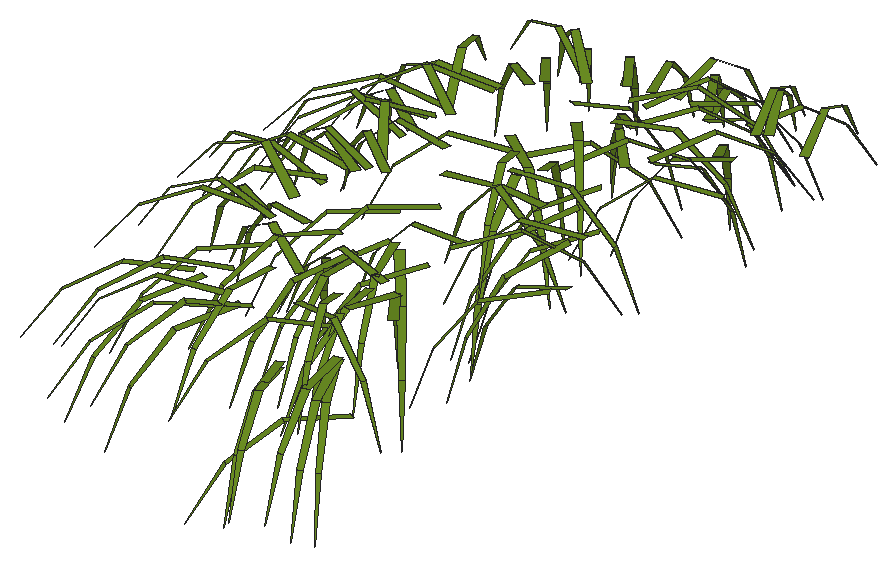
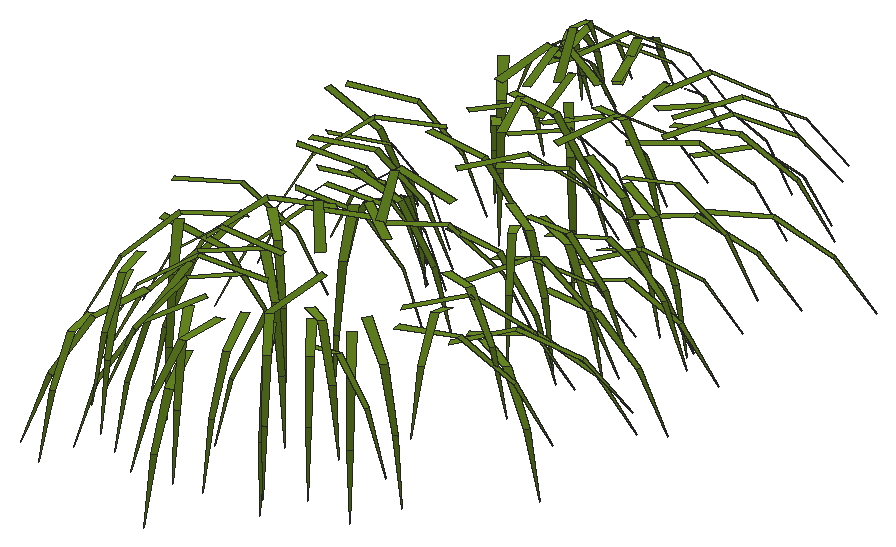
# SketchUp Ruby script. Lengths in inches.
U = 1.inch
M = Sketchup.active_model
def pt(a) = Geom::Point3d.new(a.map { |v| v * U })
def face(e, loops, mat)
  f = e.add_face(loops[0].map { |a| pt(a) })
  loops[1..].each { |l| e.add_face(l.map { |a| pt(a) }).erase! }
  f.material = f.back_material = mat if mat
  f
end
# faces: each face lists its corners as indices into pts; further lists are holes
def faces(e, pts, list, mat = nil) = list.each { |f| face(e, (f[0].is_a?(Array) ? f : [f]).map { |l| l.map { |i| pts[i] } }, mat) }
# xy, xz, yz: faces in a plane at the given z, y or x. An outline is a flat list of corners, or four numbers for a rectangle; further outlines are holes
def ring(l) = l.size == 4 ? [[l[0], l[1]], [l[2], l[1]], [l[2], l[3]], [l[0], l[3]]] : l.each_slice(2).to_a
def flat(e, list, mat, &to3) = list.each { |f| face(e, (f[0].is_a?(Array) ? f : [f]).map { |l| ring(l).map { |u, v| to3.(u, v) } }, mat) }
def xy(e, z, list, mat = nil) = flat(e, list, mat) { |x, y| [x, y, z] }
def xz(e, y, list, mat = nil) = flat(e, list, mat) { |x, z| [x, y, z] }
def yz(e, x, list, mat = nil) = flat(e, list, mat) { |y, z| [x, y, z] }
def lines(e, pts, list) = list.each { |a, b| e.add_line(pt(pts[a]), pt(pts[b])) }
# prism: a flat outline (further loops are holes) pulled along v
def prism(e, loops, v, mat = nil)
  f = face(e, loops, mat); d = Geom::Vector3d.new(v.map { |x| x * U })
  f.pushpull(f.normal.samedirection?(d) ? d.length : -d.length)
end
def box(e, o, s, mat = nil) = prism(e, [[o, [o[0] + s[0], o[1], o[2]], [o[0] + s[0], o[1] + s[1], o[2]], [o[0], o[1] + s[1], o[2]]]], [0, 0, s[2]], mat)
def at(x, y, z, deg = 0) = Geom::Transformation.translation(pt([x, y, z])) * Geom::Transformation.rotation(ORIGIN, Z_AXIS, deg.degrees)
def axes(o, x, y, z) = Geom::Transformation.new([*x, 0, *y, 0, *z, 0, *pt(o).to_a, 1])
def part(name) = M.definitions.add(name)
# library, detail: a bought-in or finely detailed component or shape, given as its bounding box
def library(name, o, s) = part(name).tap { |d| box(d.entities, o, s) }
def detail(e, o, s) = box(e.add_group.entities, o, s)
def put(e, d, t, mat = nil) = e.add_instance(d, t).tap { |i| i.material = mat if mat }
def group(e, t, mat = nil) = e.add_group.tap { |g| g.transformation = t; g.material = mat if mat }.entities
root = M.entities
M.materials.add("[0061_OliveDrab]").color = [107, 142, 35]
p = [[558.84,17.43,556.17],[558.64,17.37,556.17],[558.94,16.75,553.64],[561.49,28.35,556.17],[561.67,28.32,556.17],[561.7,29.01,553.63],
  [560.05,32.29,556.14],[560.24,32.3,556.14],[560.12,33.01,553.61],[556.33,35.38,555.85],[556.52,35.47,555.85],[555.86,36.71,553.64],
  [557.52,19.82,556.28],[557.4,20,556.28],[556.89,19.5,553.75],[556.22,25.11,556.28],[556.39,25.21,556.28],[555.97,25.77,553.75],
  [560.34,11.25,556.31],[560.17,11.11,556.31],[560.71,10.64,553.78],[560.23,14.95,556.35],[560.0625,15.05,556.35],[559.76,14.39,553.83],
  [557.125,30.02,556.3],[557.3,29.96,556.3],[557.46,30.66,553.77],[550.61,31.32,556.24],[550.78,31.45,556.24],[550.13,32.12,553.78],
  [562.33,3.99,556.375],[562.16,3.89,556.375],[562.74,3.09,553.94],[553.13,4.65,556.38],[552.93,4.75,556.38],[552.59,3.82,553.95],
  [550.63,5.69,556.26],[550.45,5.77,556.26],[550.1,4.65,553.91],[546.34,9.17,556],[546.24,9.36,556],[544.9375,8.58,553.86],
  [558.5,17.37,556.38],[558.33,17.5,556.38],[557.95,16.85,553.87],[559.33,17.32,556.42],[559.21,17.49,556.42],[558.65,16.99,553.91],
  [560.17,29.72,556.41],[560.34,29.83,556.41],[559.85,30.39,553.89],[553.38,32.92,556.3125],[553.55,33.04,556.3125],[552.94,33.75,553.86],
  [554.14,14.23,556.52],[554.29,14.37,556.52],[553.72,14.88,554.01],[560.3,15.8,556.48],[560.3125,15.99,556.48],[559.55,15.94,553.96],
  [555.68,28.9,556.47],[555.8125,29.05,556.47],[555.2,29.48,553.95],[549.85,29.7,556.44],[549.97,29.87,556.44],[549.15,30.37,553.99],
  [560.62,33.35,556.43],[560.79,33.26,556.43],[561.13,34.09,553.96],[561.81,3.6,556.51],[561.59,3.52,556.51],[562.09,2.55,554.125],
  [559.3,2.32,556.41],[559.12,2.43,556.41],[558.46,1.07,554.26],[558.97,25.82,556.75],[558.9375,26.01,556.75],[558.15,25.76,554.26],
  [546.47,26.42,556.47],[546.58,26.6,556.47],[545.28,27.31,554.3],[560.37,12.8,556.88],[560.25,12.99,556.88],[559.59,12.45,554.4],
  [545.98,20.68,556.59],[546.01,20.875,556.59],[544.54,20.99,554.42],[549.97,15.21,556.95],[550.04,15.39,556.95],[549.18,15.63,554.48],
  [553.375,32.76,556.92],[553.53,32.88,556.92],[552.78,33.73,554.55],[555.23,9,557.05],[555.03,9.07,557.05],[554.81,8.19,554.58],
  [555.34,10.51,557.05],[555.17,10.6,557.05],[554.85,9.74,554.59],[558.125,13.4,557.08],[558.3,13.53,557.08],[557.67,14.18,554.62],
  [559.74,2.57,556.85],[559.56,2.5,556.85],[560.14,1.16,554.66],[548.14,15.86,557.11],[548.24,16.04,557.11],[547.28,16.4375,554.69],
  [551.95,32.03,557.04],[552.11,32.15,557.04],[551.38,32.95,554.65],[555.03,33.72,557.02],[555.2,33.8,557.02],[554.625,34.89,554.7],
  [556.47,33.9,556.98],[556.65,34.02,556.98],[555.875,35,554.67],[561.18,3.24,557.09],[560.97,3.2,557.09],[561.35,1.98,554.79],
  [561.63,34.73,556.97],[561.85,34.7,556.97],[561.95,36.12,554.76],[557.27,10.02,557.3],[557.09,10.11,557.3],[556.72,9.24,554.85],
  [555.47,20.5,557.35],[555.51,20.72,557.35],[554.55,20.78,554.91],[546.35,22.66,557.09],[546.28,22.84,557.09],[544.93,22.23,554.92],
  [550.36,8.76,557.39],[550.24,8.9,557.39],[549.45,8.05,555.03],[547.56,15.15,557.24],[547.41,15.31,557.24],[546.48,14.29,555],
  [555,16.09,557.47],[555.01,16.28,557.47],[554.02,16.24,555.04],[560.78,35.62,557.02],[560.95,35.6875,557.02],[560.26,37.17,554.97],
  [560.04,2.46,557.18],[559.84,2.38,557.18],[560.56,0.96,555.1],[552.52,13.61,557.52],[552.4,13.77,557.52],[551.65,13.07,555.1],
  [549.33,7.52,557.36],[549.26,7.72,557.36],[547.92,7.2,555.16],[556.98,34.77,557.55],[557.18,34.8,557.55],[556.91,36.14,555.3],
  [558.04,17.8,557.84],[557.99,18,557.84],[556.97,17.66,555.44],[559.38,20.45,557.84],[559.25,20.27,557.84],[560.16,19.74,555.43],
  [561.73,21.58,557.77],[561.75,21.39,557.77],[562.78,21.56,555.37],[549.97,21.59,557.79],[550.01,21.79,557.79],[548.93,21.86,555.39],
  [559.22,10.29,557.83],[559.05,10.22,557.83],[559.58,9.23,555.45],[548.57,20.19,557.86],[548.68,20.39,557.86],[547.57,20.875,555.52],
  [545.75,18.6,557.625],[545.75,18.81,557.625],[544.04,18.68,555.63],[547.52,25.83,557.72],[547.49,26.05,557.72],[545.97,25.71,555.61],
  [557.06,27.1,557.9375],[557.2,27.24,557.9375],[556.32,28.03,555.59],[559.71,33.8125,557.84],[559.88,33.91,557.84],[559.1,35.07,555.62],
  [551.48,4.44,557.76],[551.33,4.55,557.76],[550.46,3.25,555.65],[554.38,12.95,558.11],[554.43,13.15,558.11],[553.3,13.32,555.74],
  [550.11,20.86,558.08],[550.23,21.02,558.08],[549.26,21.6,555.7],[560.01,6.83,558.12],[559.82,6.79,558.12],[560.21,5.71,555.76],
  [546.625,13.15,557.81],[546.55,13.36,557.81],[545.04,12.7,555.76],[554.09,13.77,558.17],[553.93,13.9,558.17],[553.24,12.88,555.85],
  [552.38,20.5,558.18],[552.3,20.7,558.18],[551.26,20.17,555.82],[560.04,22.71,558.16],[559.98,22.9,558.16],[558.89,22.42,555.82],
  [557.14,33.43,557.4],[557.42,33.55,557.4],[553.1,4.48,558.14],[552.92,4.59,558.14],[552.28,3.41,555.89],[555.11,5.875,558.09],
  [554.92,5.87,558.09],[555.08,4.5,555.85],[560.17,19.36,558.28],[560.16,19.14,558.28],[561.33,19.2,555.92],[562.49,26.92,558.26],
  [562.52,26.72,558.26],[563.6875,26.98,555.92],[561.45,7.63,558.28],[561.38,7.46,558.28],[562.57,7.09,555.96],[548.34,10.13,557.41],
  [548.2,10.4,557.41],[547.29,17.83,558.18],[547.27,18.05,558.18],[545.88,17.8,555.96],[559.84,32.17,558.34],[560.02,32.09,558.34],
  [560.4375,33.27,556.03],[559.39,6.9,558.37],[559.17,6.92,558.37],[559.15,5.68,556.06],[546.47,23.29,557.99],[546.39,23.48,557.99],
  [544.8,22.66,556.07],[560.31,25.19,558.4],[560.45,25.03,558.4],[561.26,25.89,556.05],[561.15,30.25,558.34],[561.3125,30.14,558.34],
  [561.98,31.33,556.09],[560.08,30.88,558.35],[560.34,30.89,558.35],[558.48,18.75,558.42],[558.2,18.66,558.42],[561.21,27.02,558.41],
  [561.46,26.97,558.41],[551.62,29.95,558.24],[551.86,30.14,558.24],[551.53,31.18,558.53],[551.68,31.34,558.53],[550.66,32.09,556.22],
  [551.4,7.46,558.04],[551.13,7.57,558.04],[553.51,9.45,558.54],[553.32,9.54,558.54],[552.88,8.28,556.28],[559.47,12.37,558.52],
  [559.23,12.17,558.52],[561.01,16.15,558.55],[560.78,16.3,558.55],[548.38,19.6,558.47],[548.43,19.79,558.47],[547.01,20.1,556.28],
  [558.6875,20.6,558.5],[558.51,20.85,558.5],[556.87,23.87,558.5],[557.11,24,558.5],[556.6,28.7,558.5],[556.85,28.61,558.5],
  [554.31,31.49,558.3],[554.54,31.64,558.3],[560.48,4.26,557.74],[560.22,4.41,557.74],[561.48,5.55,558.31],[561.23,5.41,558.31],
  [553.96,6.21,558.32],[553.67,6.35,558.32],[550.17,6.52,558.46],[550,6.67,558.46],[549.01,5.375,556.41],[558,8.09,558.63],
  [557.82,8.05,558.63],[558.19,6.69,556.42],[547.51,13.85,558.54],[547.51,14.03,558.54],[545.97,14.02,556.42],[560.56,18.11,558.6],
  [560.4,18.35,558.6],[559.44,18.49,558.56],[559.2,18.67,558.56],[562.47,18.78,558.65],[562.6,18.64,558.65],[563.52,19.67,556.42],
  [546.41,18.67,558.32],[546.5,18.875,558.32],[544.84,19.49,556.38],[548.86,19.73,558.61],[548.72,19.87,558.61],[547.76,18.78,556.42],
  [548.42,23.68,558.57],[548.33,23.87,558.57],[547.05,23.11,556.4],[560.93,28.48,558.59],[561.17,28.64,558.59],[551.18,28.62,558.41],
  [551.36,28.85,558.41],[549.74,31.49,558.39],[549.82,31.66,558.39],[548.3,32.33,556.36],[559.8,31.89,558.46],[560.04,31.76,558.46],
  [556.64,4.64,558.67],[556.48,4.74,558.67],[555.79,3.49,556.46],[561.18,5.36,558.36],[560.88,5.25,558.36],[555.08,13.07,558.67],
  [555.3,13.26,558.67],[561.78,15.68,558.65],[561.79,15.95,558.65],[548.32,25.18,557.86],[548.48,25.43,557.86],[556.74,27.87,558.64],
  [556.93,28.07,558.64],[561.34,30.23,558.74],[561.44,30.03,558.74],[562.52,30.74,556.46],[560.22,33.36,558.59],[560.39,33.43,558.59],
  [559.67,34.88,556.53],[551.68,12.85,558.85],[551.78,13.04,558.85],[550.46,13.6,556.64],[548.16,20.32,558.01],[548.2,20.6,558.01],
  [547.57,21.51,558.76],[547.58,21.7,558.76],[546.16,21.73,556.55],[548.63,25.72,558.76],[548.74,25.89,558.76],[547.39,26.6,556.62],
  [563.01,29,558.79],[563.19,28.9,558.79],[563.82,30.2,556.6],[560.53,26.08,558.84],[560.48,26.35,558.84],[559.04,4.65,558.28],
  [558.78,4.56,558.28],[558.71,18.14,559.05],[558.53,18.06,559.05],[559.25,16.82,556.85],[560.13,21.67,558.93],[559.97,21.53,558.93],
  [561.02,20.46,556.77],[561.77,13.625,558.9375],[561.61,13.89,558.9375],[550.1,22.92,559.08],[550.28,23.05,559.08],[549.34,24.17,556.89],
  [561.24,26.37,559.06],[561.42,26.24,559.06],[562.19,27.55,556.92],[554.47,31.2,558.72],[554.7,31.37,558.72],[555.87,10.5625,559.05],
  [555.59,10.67,559.05],[551.51,14.55,558.97],[551.62,14.8125,558.97],[549.46,28.73,558.94],[549.64,28.82,558.94],[548.76,30.32,556.97],
  [553.0625,30.5,558.86],[553.29,30.67,558.86],[555.79,31.875,558.72],[556.04,31.98,558.72],[557.55,32.18,558.63],[557.8,32.34,558.63],
  [561.28,32.65,558.52],[561.57,32.6,558.52],[561.62,33.41,558.16],[561.87,33.51,558.16],[560.77,5.27,558.71],[560.48,5.2,558.71],
  [556.125,12.02,559.06],[555.89,12.13,559.06],[559.11,12.01,559.08],[559.36,12.2,559.08],[549.78,14.9375,558.94],[549.91,15.1875,558.94],
  [548.48,23.42,558.42],[548.39,23.67,558.42],[559.18,4.625,558.4],[558.9,4.51,558.4],[549.2,16.63,558.66],[548.99,16.86,558.66],
  [560.26,5.98,559.35],[560.08,5.9,559.35],[560.875,4.48,557.29],[560.77,4.74,557.66],[558.15,11.54,559.25],[557.91,11.68,559.25],
  [550.69,11.29,557.33],[550.52,11.62,557.33],[561.81,6.49,557.38],[561.49,6.67,557.38],[551.4375,8.11,558.8],[551.35,8.4,558.8],
  [551.83,10.05,559.15],[551.65,10.25,559.15],[557.22,20.14,559.28],[557.28,20.44,559.28],[558.17,31.01,557.56],[558.5,31.16,557.56],
  [554.02,14.7,559.38],[553.84,14.93,559.38],[556.81,15.95,559.37],[556.82,16.23,559.37],[557.21,32.61,559.01],[557.5,32.64,559.01],
  [548.19,18.59,558.58],[548.1875,18.88,558.58],[550.5,23.74,557.59],[550.7,24.05,557.59],[562.54,31.03,557.5625],[562.84,31.15,557.5625],
  [550.65,18.59,557.66],[550.64,18.94,557.66],[549.79,26.13,559.02],[549.74,26.4375,559.02],[552.9,6.27,559],[552.6875,6.43,559],
  [558.48,12.11,559.58],[558.24,12,559.58],[548.86,13.9,558.95],[548.76,14.21,558.95],[559.93,18.21,559.61],[559.87,18.49,559.61],
  [550.75,19.91,557.85],[550.8,20.25,557.85],[557.87,21.62,559.63],[557.69,21.37,559.63],[551.87,21.24,559.57],[551.91,21.52,559.57],
  [559.83,21.47,559.58],[559.85,21.21,559.58],[560.76,31.88,559.28],[561.01,32.03,559.28],[558.21,7.02,557.92],[557.87,6.875,557.92],
  [550.33,19.15,559.49],[550.49,19.42,559.49],[558.42,25.62,559.62],[558.62,25.81,559.62],[552.41,9.87,558.35],[552.08,10,558.35],
  [550.82,16.62,558.04],[550.98,16.97,558.04],[548.79,17.91,559.15],[548.66,17.62,559.15],[548.75,24.25,558.88],[548.63,24.53,558.88],
  [550.91,24.3,557.97],[550.8,24.61,557.97],[551.02,25.22,557.98],[550.87,25.56,557.98],[554.33,6.3125,559.56],[554.07,6.48,559.56],
  [558.18,7.13,558.11],[557.86,7.01,558.11],[555.04,8.04,559.57],[554.78,8.03,559.57],[559.53,8.79,559.81],[559.27,8.72,559.81],
  [556.32,12.43,559.8],[556.39,12.7,559.8],[551.09,18.37,558.14],[550.84,18.64,558.14],[551.71,19.66,559.78],[551.87,19.89,559.78],
  [555.41,15.36,559.78],[555.19,15.54,559.78],[549.52,18,559.55],[549.49,18.31,559.55],[554.29,21.2,559.84],[554.18,21.48,559.84],
  [561.99,23.34,559.81],[561.9,23.6,559.81],[553.17,27.89,558.73],[553.46,28.12,558.73],[560.2,7.82,558.65],[559.9,7.65,558.65],
  [555.14,8.52,558.75],[554.79,8.69,558.75],[559.5,8.45,559.83],[559.4,8.2,559.83],[558.13,19.5,559.92],[558.12,19.18,559.92],
  [560.44,26.69,559.88],[560.48,26.41,559.88],[559.92,28.46,559.82],[560.15,28.31,559.82],[555.72,29.34,558.82],[556,29.53,558.82],
  [558.94,30.25,559.89],[559.19,30.14,559.89],[560.29,7.8125,558.65],[559.92,7.67,558.65],[559.65,8.99,559.94],[559.35,9.02,559.94],
  [551.29,14.74,558.39],[551.16,15.11,558.39],[557.81,21.04,559.5],[557.46,20.93,559.5],[558.73,23.86,560.01],[558.93,23.625,560.01],
  [560.75,24.67,559.5],[561.07,24.62,559.5],[553.2,27.02,558.96],[553.42,27.31,558.96],[560.15,28.45,559.34],[560.48,28.47,559.34],
  [551.88,30.35,559.4],[552,30.59,559.4],[554.47,8.3125,558.51],[554.21,8.51,558.51],[551.78,8.27,559.58],[551.54,8.48,559.58],
  [554.43,11.43,560.01],[554.15,11.55,560.01],[557.93,14.26,559.5],[557.64,14.01,559.5],[549.83,13.7,559.76],[549.84,13.96,559.76],
  [562.32,18.22,559.5],[562.04,18.39,559.5],[550.53,18.9375,559.8125],[550.61,19.2,559.8125],[560.68,21.98,559.5],[560.46,22.29,559.5],
  [558.02,21.73,559.5],[558.32,21.9,559.5],[555.74,26.41,559.47],[556.04,26.3,559.47],[554.04,29.21,558.45],[554.19,29.51,558.45],
  [558.5625,29.64,558.98],[558.86,29.48,558.98],[553.13,29.72,560.01],[553.33,29.94,560.01],[560.85,30.06,558.66],[561.22,30,558.66],
  [553.95,8.83,558.63],[553.85,9.19,558.63],[557.59,10.28,560.02],[557.34,10.23,560.02],[564.26,15.52,559.5],[564.27,15.85,559.5],
  [562.62,19.47,559.5],[562.42,19.76,559.5],[560.99,20.39,559.5],[560.7,20.62,559.5],[550.51,21.33,559.87],[550.33,21.52,559.87],
  [550.5,24.68,559.82],[550.37,24.94,559.82],[558.54,26.17,559.5],[558.59,26.22,559.5],[558.77,26.42,559.5],[562.26,26.41,559.5],
  [562.56,26.61,559.5],[558.97,29.97,558.64],[559.27,30.16,558.64],[561.1,31.18,559.77],[561.34,31.28,559.77],[557.9,6.53,559.98],
  [557.68,6.67,559.98],[560.24,7.84,558.69],[559.88,7.76,558.69],[556.6875,11.17,559.5],[556.95,11.4,559.5],[560.85,17.26,560.06],
  [561.04,17.07,560.06],[551.61,24.38,558.7],[551.91,24.53,558.7],[550.8,26.63,559.8125],[550.55,26.51,559.8125],[552.37,26.48,558.7],
  [552.31,26.86,558.7],[559.39,29.22,560.1875],[559.54,28.94,560.1875],[556,29.08,558.99],[556.28,29.29,558.99],[556.81,29.46,558.89],
  [557.11,29.6,558.89],[557.5,30.02,558.65],[557.85,30.07,558.65],[553.68,11.77,560.16],[553.82,12.04,560.16],[549.85,21.26,560.04],
  [549.87,21.54,560.04],[550.59,24.47,559.98],[550.74,24.71,559.98],[563.03,26.53,559.5],[562.97,26.87,559.5],[561.84,27.0625,560.125],
  [562.1,26.91,560.125],[555.72,8.43,558.88],[555.41,8.63,558.88],[553.48,10.14,558.875],[553.19,10.4,558.875],[563.97,14.95,559.5],
  [563.76,15.28,559.5],[552.07,13.67,558.98],[552.24,13.97,558.98],[552.07,18.21,558.94],[552.03,18.59,558.94],[558.68,23.45,560.18],
  [558.45,23.26,560.18],[554.62,28.39,558.97],[554.9,28.6,558.97],[562.03,29.62,558.88],[562.33,29.79,558.88],[553.9,13.5625,559.42],
  [554.03,13.89,559.42],[557.75,20.22,560.34],[557.5,20.1,560.34],[552.29,23.06,559.03],[552.0625,23.3,559.03],[552.75,25.78,559.03],
  [552.59,26.1,559.03],[560.65,9.92,559.48],[560.96,10.15,559.48],[553.77,11.81,559.26],[553.55,12.05,559.26],[556.82,12.97,559.5],
  [556.48,13.1,559.5],[557.3,14.32,559.5],[557.2,14.37,559.5],[557.01,14.47,559.5],[552.36,13.55,559.09],[552.38,13.87,559.09],
  [552.29,21.01,559.11],[552.32,21.35,559.11],[551.42,21.01,560.3],[551.67,21.19,560.3],[559.88,24.48,560.27],[560.14,24.3,560.27],
  [559.29,8.63,559.22],[559.01,8.8,559.22],[559.4375,13.82,559.5],[559.14,13.98,559.5],[552.6,17.84,559.24],[552.79,18.17,559.24],
  [554.98,28.05,559.18],[555.23,28.32,559.18],[554.95,10.65,559.28],[554.63,10.63,559.28],[557.12,9.41,559.26],[557,9.11,559.26],
  [553,18.19,559.31],[553.09,18.51,559.31],[552.81,19.02,559.29],[553.12,19.25,559.29],[559.79,19.625,559.5],[559.85,19.99,559.5],
  [552.73,23.125,559.26],[552.91,23.42,559.26],[562.08,28.8,559.26],[562.375,28.93,559.26],[559.25,8.17,560.4],[559,8.05,560.4],
  [555.89,10.58,559.39],[556.0625,10.91,559.39],[556.125,16.26,559.5],[555.9,16.55,559.5],[559.42,15.78,559.5],[559.44,16.12,559.5],
  [557.18,28.05,559.38],[557.36,27.72,559.38],[557.87,27.91,559.41],[558.17,27.77,559.41],[558.22,10.39,559.47],[557.91,10.24,559.47],
  [558.89,11.32,559.5],[558.58,11.23,559.5],[559.95,11.5625,559.5],[559.58,11.6,559.5],[557.11,12.8,559.5],[556.8,12.74,559.5],
  [555.49,13.77,559.5],[555.15,13.92,559.5],[558.84,11.77,559.5],[558.93,12.11,559.5],[557.47,14.53,559.5],[557.18,14.4,559.5],
  [559,15.49,559.5],[559.22,15.26,559.5],[557.07,17.38,559.5],[556.8,17.59,559.5],[553.8,18.11,559.48],[554,18.39,559.48],
  [562.49,18.78,559.5],[562.41,19.12,559.5],[555.55,19.65,559.5],[555.53,19.26,559.5],[556.6875,22.47,559.5],[556.6,22.43,559.5],
  [556.38,22.32,559.5],[554.45,20.79,559.5],[554.51,21.14,559.5],[557.21,21.3125,559.5],[557.24,20.99,559.5],[556.72,22.12,559.5],
  [556.59,22.46,559.5],[555.78,23.21,559.5],[555.56,22.9,559.5],[556.77,22.18,559.5],[557.02,21.89,559.5],[558.43,22.43,559.5],
  [558.74,22.22,559.5],[557.07,25.41,559.5],[556.79,25.17,559.5],[564.46,24.16,559.5],[564.35,24.48,559.5],[560.2,23.69,559.5],
  [560.45,23.93,559.5],[560.54,24.87,559.5],[560.86,24.6875,559.5],[557.86,26.38,559.5],[557.91,26.04,559.5],[558.46,26.3,559.5],
  [558.74,26.11,559.5]]
faces(root,p,[[0,1,2],[3,4,5],[6,7,8],[9,10,11],[12,13,14],[15,16,17],[18,19,20],[21,22,23],
  [24,25,26],[27,28,29],[30,31,32],[33,34,35],[36,37,38],[39,40,41],[42,43,44],[45,46,47],
  [48,49,50],[51,52,53],[54,55,56],[57,58,59],[60,61,62],[63,64,65],[66,67,68],[69,70,71],
  [72,73,74],[75,76,77],[78,79,80],[81,82,83],[84,85,86],[87,88,89],[90,91,92],[93,94,95],
  [96,97,98],[99,100,101],[102,103,104],[105,106,107],[108,109,110],[111,112,113],[114,115,116],[117,118,119],
  [120,121,122],[123,124,125],[126,127,128],[129,130,131],[132,133,134],[135,136,137],[138,139,140],[141,142,143],
  [144,145,146],[147,148,149],[150,151,152],[153,154,155],[156,157,158],[159,160,161],[162,163,164],[165,166,167],
  [168,169,170],[171,172,173],[174,175,176],[177,178,179],[180,181,182],[183,184,185],[186,187,188],[189,190,191],
  [192,193,194],[195,196,197],[198,199,200],[201,202,203],[204,205,206],[207,208,209],[210,211,10,9],[212,213,214],
  [215,216,217],[218,219,220],[221,222,223],[224,225,226],[227,228,40,39],[229,230,231],[232,233,234],[235,236,237],
  [238,239,240],[241,242,243],[244,245,246],[247,248,7,6],[249,250,1,0],[251,252,4,3],[253,254,28,27],[255,256,257],
  [258,259,37,36],[260,261,262],[263,264,19,18],[265,266,22,21],[267,268,269],[270,271,13,12],[272,273,16,15],[274,275,25,24],
  [276,277,52,51],[278,279,73,72],[280,281,31,30],[282,283,34,33],[284,285,286],[287,288,289],[290,291,292],[293,294,46,45],
  [295,296,43,42],[297,298,299],[300,301,302],[303,304,305],[306,307,308],[309,310,49,48],[311,312,64,63],[313,314,315],
  [316,317,67,66],[318,319,320],[321,322,70,69],[323,324,55,54],[325,326,58,57],[327,328,79,78],[329,330,61,60],[331,332,333],
  [334,335,336],[337,338,339],[340,341,85,84],[342,343,344],[345,346,347],[348,349,350],[351,352,76,75],[353,354,103,102],
  [355,356,357],[358,359,360],[361,362,82,81],[363,364,365],[366,367,368],[369,370,91,90],[371,372,94,93],[373,374,88,87],
  [375,376,377],[378,379,109,108],[380,381,112,111],[382,383,115,114],[384,385,121,120],[386,387,142,141],[388,389,118,117],[390,391,97,96],
  [392,393,100,99],[394,395,106,105],[396,397,130,129],[398,399,145,144],[400,401,136,135],[402,403,404,405],[406,407,124,123],[408,409,228,227],
  [410,411,279,278,405],[412,413,151,150],[414,415,133,132],[416,417,127,126],[418,419,211,210],[420,421,148,147],[422,423,139,138],[424,425,154,153],
  [426,427,175,174],[428,429,328,327],[430,431,387,386],[432,433,427,426],[434,435,178,177],[436,437,187,186],[438,439,169,168],[440,441,199,198],
  [442,443,157,156],[444,445,341,340],[446,447,160,159],[448,449,166,165],[450,451,163,162],[452,453,184,183],[454,455,399,398],[456,457,172,171],
  [458,459,181,180],[460,461,259,258],[462,463,464,465],[466,467,239,238],[468,469,397,396],[470,471,467,466],[472,473,213,212],[474,475,354,353],
  [476,477,216,215],[478,479,196,195],[480,481,190,189],[482,483,401,400],[484,485,193,192],[486,487,202,201],[488,489,230,229],[490,491,205,204],
  [492,493,208,207],[494,495,254,253],[496,497,281,280],[498,499,283,282],[500,501,225,224],[465,464,301,300],[502,503,219,218],[504,505,222,221],
  [506,507,245,244],[508,509,277,276],[510,511,233,232],[512,513,322,321],[514,515,236,235],[516,517,441,440],[518,519,250,249],[520,521,242,241],
  [522,523,252,251],[524,525,312,311],[526,527,248,247],[528,529,314,313],[530,531,437,436],[532,533,285,284],[534,535,261,260],[536,537,264,263],
  [538,539,291,290],[540,541,266,265],[542,543,268,267],[544,545,271,270],[546,547,273,272],[548,549,275,274],[550,551,529,528],[552,553,317,316],
  [554,555,256,255],[556,557,385,384],[558,559,413,412],[560,561,288,287],[562,563,326,325],[564,565,294,293],[566,567,296,295],[568,569,304,303],
  [570,571,307,306],[572,573,574,330,329],[575,576,310,309],[577,578,383,382],[579,580,335,334],[581,582,319,318],[583,584,389,388],[585,586,324,323],
  [587,588,298,297],[589,590,591,592],[593,594,435,434],[595,596,332,331],[597,598,370,369],[599,600,381,380],[601,602,425,424],[603,604,338,337],
  [605,606,343,342],[607,608,346,345],[609,610,352,351],[611,612,349,348],[613,614,473,472],[615,616,533,532],[617,618,362,361],[619,620,395,394],
  [621,622,489,488],[623,624,359,358],[592,591,376,375],[625,626,379,378],[627,628,453,452],[629,630,374,373],[631,632,356,355],[633,634,569,568],
  [635,636,571,570],[637,638,393,392],[639,640,415,414],[641,642,372,371],[643,644,645,391,390],[646,647,539,538],[648,649,606,605],[650,651,364,363],
  [652,653,367,366],[654,655,582,581],[656,657,407,406],[658,659,457,456],[660,661,555,554],[662,663,477,476],[664,665,501,500],[666,667,543,542],
  [668,669,651,650],[670,671,417,416],[672,673,608,607],[674,675,580,579],[676,677,403,402],[678,679,604,603],[680,681,421,420],[682,683,423,422],
  [684,685,596,595],[686,687,511,510],[688,689,677,676],[690,691,479,478],[692,693,515,514],[694,695,561,560],[696,697,535,534],[698,699,481,480],
  [700,701,644,439,438],[702,703,588,587],[704,705,487,486],[706,707,485,484],[708,709,443,442],[710,711,503,502],[712,713,714,632,631],[715,716,449,448],
  [717,718,451,450],[719,713,720,491,490],[721,722,447,446],[723,724,521,520],[725,726,653,652],[727,728,624,623],[729,730,493,492],[731,732,459,458],
  [733,734,612,611],[735,736,505,504],[737,573,738,507,506]],"[0061_OliveDrab]")
